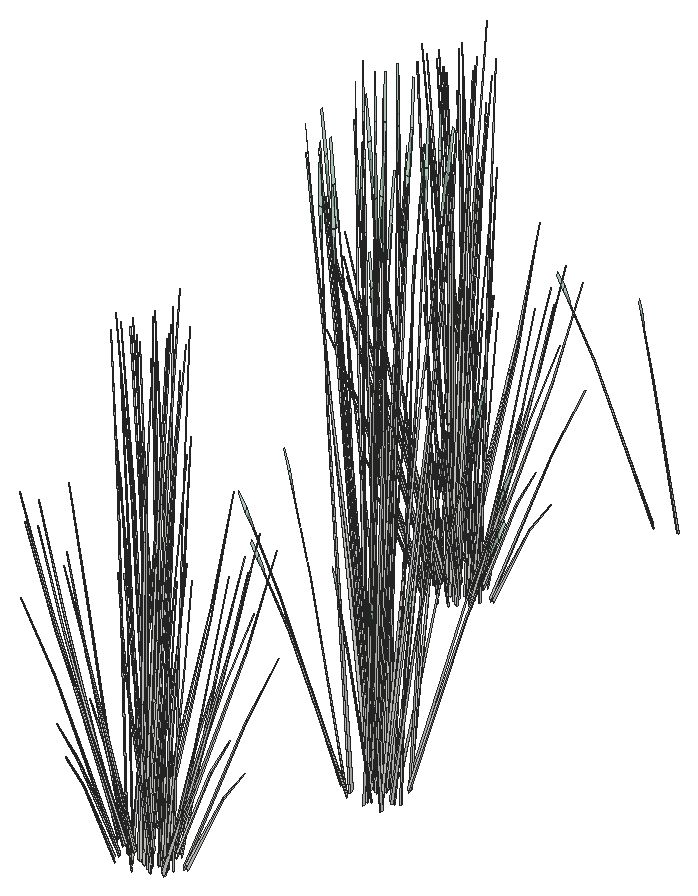
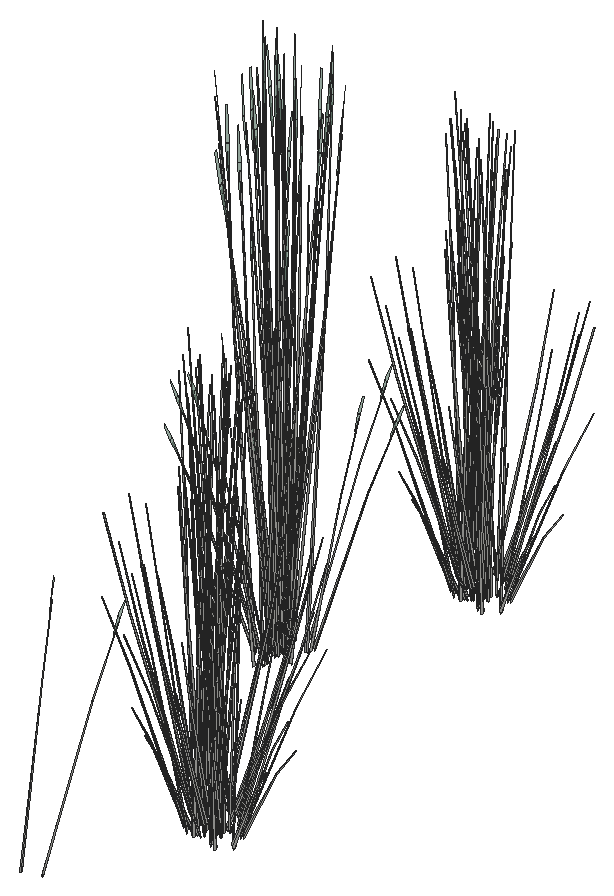
# SketchUp Ruby script. Lengths in inches.
U = 1.inch
M = Sketchup.active_model
def pt(a) = Geom::Point3d.new(a.map { |v| v * U })
def face(e, loops, mat)
  f = e.add_face(loops[0].map { |a| pt(a) })
  loops[1..].each { |l| e.add_face(l.map { |a| pt(a) }).erase! }
  f.material = f.back_material = mat if mat
  f
end
# faces: each face lists its corners as indices into pts; further lists are holes
def faces(e, pts, list, mat = nil) = list.each { |f| face(e, (f[0].is_a?(Array) ? f : [f]).map { |l| l.map { |i| pts[i] } }, mat) }
# xy, xz, yz: faces in a plane at the given z, y or x. An outline is a flat list of corners, or four numbers for a rectangle; further outlines are holes
def ring(l) = l.size == 4 ? [[l[0], l[1]], [l[2], l[1]], [l[2], l[3]], [l[0], l[3]]] : l.each_slice(2).to_a
def flat(e, list, mat, &to3) = list.each { |f| face(e, (f[0].is_a?(Array) ? f : [f]).map { |l| ring(l).map { |u, v| to3.(u, v) } }, mat) }
def xy(e, z, list, mat = nil) = flat(e, list, mat) { |x, y| [x, y, z] }
def xz(e, y, list, mat = nil) = flat(e, list, mat) { |x, z| [x, y, z] }
def yz(e, x, list, mat = nil) = flat(e, list, mat) { |y, z| [x, y, z] }
def lines(e, pts, list) = list.each { |a, b| e.add_line(pt(pts[a]), pt(pts[b])) }
# prism: a flat outline (further loops are holes) pulled along v
def prism(e, loops, v, mat = nil)
  f = face(e, loops, mat); d = Geom::Vector3d.new(v.map { |x| x * U })
  f.pushpull(f.normal.samedirection?(d) ? d.length : -d.length)
end
def box(e, o, s, mat = nil) = prism(e, [[o, [o[0] + s[0], o[1], o[2]], [o[0] + s[0], o[1] + s[1], o[2]], [o[0], o[1] + s[1], o[2]]]], [0, 0, s[2]], mat)
def at(x, y, z, deg = 0) = Geom::Transformation.translation(pt([x, y, z])) * Geom::Transformation.rotation(ORIGIN, Z_AXIS, deg.degrees)
def axes(o, x, y, z) = Geom::Transformation.new([*x, 0, *y, 0, *z, 0, *pt(o).to_a, 1])
def part(name) = M.definitions.add(name)
# library, detail: a bought-in or finely detailed component or shape, given as its bounding box
def library(name, o, s) = part(name).tap { |d| box(d.entities, o, s) }
def detail(e, o, s) = box(e.add_group.entities, o, s)
def put(e, d, t, mat = nil) = e.add_instance(d, t).tap { |i| i.material = mat if mat }
def group(e, t, mat = nil) = e.add_group.tap { |g| g.transformation = t; g.material = mat if mat }.entities
root = M.entities
M.materials.add("LightPink_Translucent").color = [175, 214, 192]
M.materials["LightPink_Translucent"].alpha = 0.75
c1 = part("blade")
p = [[2.15,0.21,22],[0,0.17,0],[0.09,0.45,0],[2.18,0.31,22],[2.29,0.31,22],[0.38,0.45,0],
  [2.48,0.24,33],[2.49,0.24,33],[2.48,0.22,33]]
faces(c1.entities,p,[[0,1,2,3],[4,5,2,3],[6,3,4,7],[8,0,3,6]])
c2 = part("blade with seeds\#1")
put(c2.entities,c1,at(0,0,0))
c3 = part("seeds")
p = [[0.3,-0.1,1.38],[-0.01,-0.03,1.59],[-0.01,-0.03,0.03],[0.14,-0.07,-0.07],[0.29,-0.03,3],[0.15,0.01,3.11]]
faces(c3.entities,p,[[0,1,2,3],[1,0,4,5]],"LightPink_Translucent")
c4 = part("blade with seeds")
put(c4.entities,c1,at(0,0,0))
put(c4.entities,c3,axes([2.4,0.25,30.99],[1.5799,-0.05474,1.17369],[-0.12525,1.92788,0.29478],[-0.07173,-0.02425,1.56792]))
put(root,c2,axes([494.86,352.5,140.9],[0.01294,-0.35246,-0.58282],[0.54471,0.02367,0.07033],[0.05748,-0.14932,0.82446]))
put(root,c2,axes([493.99,351.32,139.08],[0.06377,0.2222,0.94226],[-0.35378,-0.12306,0.69231],[0.03807,-0.11377,0.20754]))
put(root,c2,axes([493.69,352.14,140.65],[-0.48869,-0.09552,-0.41919],[0.16751,-0.3275,-0.3247],[-0.04481,-0.13186,0.80208]))
put(root,c2,axes([494.75,352.39,140.65],[-0.35588,-0.25603,-0.41919],[0.37594,-0.22422,-0.3247],[0.05415,-0.13008,0.80208]))
put(root,c2,axes([492.18,351.58,139.08],[0.25932,0.13262,0.94226],[-0.37767,0.07972,0.69231],[-0.08081,-0.10192,0.20754]))
put(root,c2,axes([492.8,352.29,140.9],[-0.4239,-0.18418,-0.58282],[0.30126,-0.32274,0.07033],[-0.15358,-0.10997,0.82446]))
put(root,c2,axes([492.6,352.3,140.65],[-0.49056,0.09058,-0.41919],[-0.08581,-0.34303,-0.3247],[-0.13176,-0.0983,0.80208]))
put(root,c2,axes([495.49,352.98,140.65],[-0.12771,-0.34793,-0.41919],[0.48364,-0.06086,-0.3247],[0.1386,-0.09345,0.80208]))
put(root,c2,axes([495.5,353.12,140.9],[0.25968,-0.30066,-0.58282],[0.45504,0.21367,0.07033],[0.15505,-0.10893,0.82446]))
put(root,c2,axes([495.875,352.84,138.9375],[-0.1776,-0.01129,1.17311],[-0.18194,-0.30276,-0.25229],[0.21818,-0.08565,0.50157]))
put(root,c2,axes([496.08,352.28,139.08],[-0.16559,0.19397,0.94226],[-0.14233,-0.26061,0.69231],[0.13676,-0.0653,0.20754]))
put(root,c2,axes([491.54,352.84,138.9375],[0.09706,0.10609,1.17311],[-0.22366,0.28837,-0.25229],[-0.22965,-0.06892,0.50157]))
put(root,c2,axes([491.9375,352.74,140.9],[-0.49695,-0.00917,-0.58282],[0.03338,-0.38634,0.07033],[-0.21053,-0.04077,0.82446]))
put(root,c2,axes([491.77,352.82,140.65],[-0.36098,0.25241,-0.41919],[-0.31614,-0.26664,-0.3247],[-0.18341,-0.0384,0.80208]))
put(root,c2,axes([493.38,353.64,138.81],[0.56014,0.18468,0.19741],[-0.26958,0.38374,0.41019],[0,-0.08846,1.31701]))
put(root,c2,axes([490.96,353.16,139.08],[0.31739,-0.02727,0.94226],[-0.20133,0.24024,0.69231],[-0.15684,-0.03604,0.20754]))
put(root,c2,axes([493.2,353.38,139.04],[-0.53984,0.02352,0.36702],[-0.04882,-0.39046,-0.17663],[0.09664,-0.03957,1.17838]))
put(root,c2,axes([491.81,353.66,138.85],[0,0.38104,0.40731],[-0.5562,0,0],[0,-0.08679,1.29208]))
put(root,c2,axes([493.18,353.52,138.75],[0.21614,0.42608,0.37535],[-0.61757,0.14817,0.14729],[0.00755,-0.07829,1.30318]))
put(root,c2,axes([495.71,353.75,140.65],[0.13468,-0.34661,-0.41919],[0.46175,0.1188,-0.3247],[0.18591,-0.03178,0.80208]))
put(root,c2,axes([494.71,352.54,138.85],[-0.46527,-0.19052,0.40731],[0.2781,-0.34163,0],[0.10597,0.04339,1.29208]))
put(root,c2,axes([493.07,353.85,139.04],[-0.2412,0.34335,0.36702],[-0.50118,-0.16524,-0.17663],[0,-0.07915,1.17838]))
put(root,c2,axes([493.67,353.28,138.75],[-0.41219,0.3458,0.37535],[-0.4897,-0.30525,0.14729],[0.09937,-0.03451,1.30318]))
put(root,c2,axes([492.95,352.71,138.84],[-0.14361,0.37869,0.14473],[-0.52552,-0.10717,0.28783],[0.09078,-0.00184,1.3159]))
put(root,c2,axes([495.625,353.875,140.9],[0.43684,-0.16829,-0.58282],[0.24345,0.34641,0.07033],[0.21107,-0.03935,0.82446]))
put(root,c2,axes([494.05,353.13,138.96],[0.0959,-0.34006,0.11878],[0.46856,0.05903,-0.33919],[0.08527,0.03492,1.03975]))
put(root,c2,axes([493.85,353.22,139.04],[-0.29864,-0.31983,0.36702],[0.45236,-0.22522,-0.17663],[0.09664,0.03957,1.17838]))
put(root,c2,axes([493.24,353.9375,138.75],[0.62833,0.08028,0.37535],[-0.12787,0.45342,0.14729],[-0.09182,-0.04378,1.30318]))
put(root,c2,axes([494.54,352.73,138.84],[-0.5342,0.10113,0.14473],[-0.13191,-0.37638,0.28783],[0.04764,0.05484,1.3159]))
put(root,c2,axes([492.9,354.66,138.84],[0.5342,-0.10113,0.14473],[0.13191,0.37638,0.28783],[-0.04764,-0.05484,1.3159]))
put(root,c2,axes([494.2,353.45,138.77],[-0.62833,-0.08028,0.4036],[0.12787,-0.45342,0.15838],[0.09182,0.04378,1.40127]))
put(root,c2,axes([493.39,354.26,138.96],[-0.0959,0.34006,0.11878],[-0.46856,-0.05903,-0.33919],[-0.08527,-0.03492,1.03975]))
put(root,c2,axes([494.37,353.82,138.63],[0.34702,0.24613,0],[-0.34702,0.24613,0],[0,0,1.38858]))
put(root,c2,axes([495.31,353.72,138.84],[-0.39059,-0.27756,0.14473],[0.39362,-0.26921,0.28783],[-0.04314,0.05668,1.3159]))
put(root,c2,axes([496.87,353.97,139.08],[-0.30716,0.06291,0.94226],[0.14458,-0.25998,0.69231],[0.16295,0.01779,0.20754]))
put(root,c2,axes([494.49,354.68,138.84],[0.14361,-0.37869,0.14473],[0.52552,0.10717,0.28783],[-0.09078,0.00184,1.3159]))
put(root,c2,axes([494.37,353.53,139.04],[0.2412,-0.34335,0.36702],[0.50118,0.16524,-0.17663],[0,0.07915,1.17838]))
put(root,c2,axes([492.73,354.85,138.85],[0.46527,0.19052,0.40731],[-0.2781,0.34163,0],[-0.10597,-0.04339,1.29208]))
put(root,c2,axes([491.42,353.57,140.65],[-0.13468,0.34661,-0.41919],[-0.46175,-0.1188,-0.3247],[-0.18591,0.03178,0.80208]))
put(root,c2,axes([495.63,353.73,138.85],[0,-0.38104,0.40731],[0.5562,0,0],[0,0.08679,1.29208]))
put(root,c2,axes([494.58,353.61,138.96],[0.46318,-0.11112,0.11878],[0.1622,0.31732,-0.33919],[0,0.06984,1.03975]))
put(root,c2,axes([494.24,354.01,139.04],[0.53984,-0.02352,0.36702],[0.04882,0.39046,-0.17663],[-0.09664,0.03957,1.17838]))
put(root,c2,axes([496.3,354.39,138.9375],[-0.11973,-0.09372,1.17311],[0.15578,-0.31002,-0.25229],[0.24224,0.042,0.50157]))
put(root,c2,axes([494.25,354.18,138.96],[0.36728,0.22894,0.11878],[-0.30636,0.25829,-0.33919],[-0.08527,0.03492,1.03975]))
put(root,c2,axes([495.2,354.58,140.9],[0.49695,0.00917,-0.58282],[-0.03338,0.38634,0.07033],[0.21053,0.04077,0.82446]))
put(root,c2,axes([494.64,354.88,138.85],[0.46527,-0.19052,0.40731],[0.2781,0.34163,0],[-0.10597,0.04339,1.29208]))
put(root,c2,axes([490.87,354.38,138.9375],[0.17277,0.03128,1.17311],[0.11135,0.3195,-0.25229],[-0.23468,0.05981,0.50157]))
put(root,c2,axes([490.51,355.05,139.08],[0.20718,-0.1727,0.94226],[0.08175,0.27339,0.69231],[-0.14972,0.04895,0.20754]))
put(root,c2,axes([495.16,354.87,139.08],[-0.27991,-0.10956,0.94226],[0.36143,-0.11132,0.69231],[0.09749,0.0943,0.20754]))
put(root,c2,axes([491.65,354.34,140.65],[0.12771,0.34793,-0.41919],[-0.48364,0.06086,-0.3247],[-0.1386,0.09345,0.80208]))
put(root,c2,axes([494.48,353.64,139.14],[-0.01358,-0.35877,1.15892],[0.61462,0.093,0.4907],[-0.14537,0.19631,1.09393]))
put(root,c2,axes([494.53,355.02,140.65],[0.49056,-0.09058,-0.41919],[0.08581,0.34303,-0.3247],[0.13176,0.0983,0.80208]))
put(root,c2,axes([495.21,355.37,139],[-0.31879,-0.01195,0.86186],[0.21053,-0.25381,0.47585],[0.12594,0.09017,0.67605]))
put(root,c2,axes([494.17,354.75,138.9375],[0.00877,-0.12631,1.17311],[0.41923,-0.14109,-0.25229],[0.12942,0.15118,0.50157]))
put(root,c2,axes([492.27,355.81,139.08],[-0.01287,-0.22657,0.94226],[0.32149,0.1616,0.69231],[-0.06323,0.10799,0.20754]))
put(root,c2,axes([493.44,355.18,140.65],[0.48869,0.09552,-0.41919],[-0.16751,0.3275,-0.3247],[0.04481,0.13186,0.80208]))
put(root,c2,axes([492,355.32,139.13],[0.45162,-0.06748,0.05338],[0.10383,0.27185,-0.708],[-0.02863,0.13761,0.63462]))
put(root,c2,axes([493.26,355.12,140.9],[0.23727,0.30983,-0.58282],[-0.48842,0.17267,0.07033],[0.05548,0.1497,0.82446]))
put(root,c2,axes([491.89,355.61,138.9375],[0.15688,-0.06011,1.17311],[0.38733,0.18125,-0.25229],[-0.11528,0.15683,0.50157]))
put(root,c4,axes([499.62,368.8,139.62],[-0.03656,0.1661,1.30132],[-0.37341,0.10705,-0.27986],[-0.0699,-0.22562,0.55638]))
put(root,c4,axes([501.43,369.44,139.62],[-0.12399,0.09331,1.30132],[-0.33702,-0.21502,-0.27986],[0.08055,-0.22079,0.55638]))
put(root,c4,axes([498.84,370.33,139.42],[-0.44625,-0.29882,0],[0.24886,-0.49993,-0.46963],[0.05668,-0.11386,1.48977]))
put(root,c4,axes([498.19,369.78,139.62],[0.07025,0.15082,1.30132],[-0.21183,0.37238,-0.27986],[-0.18329,-0.11083,0.55638]))
put(root,c4,axes([502.2,369.57,139.2],[-0.36364,-0.13787,-0.03542],[0.11186,-0.42434,-0.16061],[0.05948,-0.06443,0.52975]))
put(root,c4,axes([502.65,370.2,139.62],[-0.14568,-0.02894,1.30132],[-0.12195,-0.4231,-0.27986],[0.1883,-0.0989,0.55638]))
put(root,c4,axes([499.89,371.27,139.69],[-0.29566,-0.48255,-0.26477],[0.41776,-0.32089,-0.45502],[0.04243,-0.11906,1.45334]))
put(root,c4,axes([500.54,369.34,139.42],[0,-0.59763,0],[0.49772,0,-0.46963],[0.11336,0,1.48977]))
put(root,c4,axes([500.67,369.8,139.39],[-0.37441,-0.44456,0.27988],[0.37047,-0.44483,-0.33208],[0.10632,-0.01552,1.50045]))
put(root,c4,axes([499.76,371.8125,139.51],[0.35844,-0.4667,-0.22925],[0.40249,0.39271,0.50168],[-0.04193,-0.12567,1.53076]))
put(root,c4,axes([499.89,371.01,139.48],[0.5277,0.12668,-0.2132],[-0.09198,0.60063,0.46656],[0.07287,-0.10495,1.42361]))
put(root,c4,axes([499.76,371.23,139.65],[-0.39744,-0.0922,0.13176],[0.06899,-0.45047,-0.37626],[0.04081,-0.08198,1.15337]))
put(root,c4,axes([498.77,372.15,139.26],[0.44781,-0.29509,-0.04679],[0.24886,0.49993,0.46963],[-0.04264,-0.12319,1.48904]))
put(root,c4,axes([500.36,370.87,139.69],[0.21249,-0.53825,-0.26477],[0.44849,0.25917,-0.45502],[0.11011,-0.01692,1.45334]))
put(root,c4,axes([498.53,369.89,139.83],[0.07886,0.43418,0.05922],[-0.31771,0.09982,-0.78537],[-0.16083,-0.02753,0.70398]))
put(root,c4,axes([499.96,371.94,139.69],[-0.50815,0.05569,-0.26477],[-0.03072,-0.58006,-0.45502],[-0.06769,-0.10214,1.45334]))
put(root,c4,axes([502.66,371.21,139.2],[-0.25548,-0.33028,-0.03542],[0.27981,-0.30262,-0.16061],[0.07928,-0.02131,0.52975]))
put(root,c4,axes([500.14,371.08,139.41],[-0.09383,0.60408,0.41637],[-0.52992,-0.12294,0.16339],[0.05117,-0.08828,1.44559]))
put(root,c4,axes([499.22,371.41,139.26],[0.19993,-0.48183,0],[0.41543,0.23189,0],[0,0,1.48063]))
put(root,c4,axes([498.72,372.53,139.42],[-0.44625,0.29882,0],[-0.24886,-0.49993,-0.46963],[-0.05668,-0.11386,1.48977]))
put(root,c4,axes([499.86,372.05,139.65],[-0.26757,0.3531,0.13176],[-0.30187,-0.29453,-0.37626],[-0.04081,-0.08198,1.15337]))
put(root,c4,axes([500.1875,371.92,139.36],[0.3833,-0.44456,-0.05579],[0.38354,0.44483,0],[0.01339,-0.01552,1.5977]))
put(root,c4,axes([499,372.17,139.39],[-0.14475,0.59835,0.27988],[-0.51739,-0.14969,-0.33208],[-0.06475,-0.09903,1.50045]))
put(root,c4,axes([500.63,371.03,139.41],[-0.49797,0.2078,0.41637],[-0.17316,-0.59373,0.16339],[0.0915,0.00726,1.44559]))
put(root,c4,axes([499.4,371.52,139.27],[0.38394,-0.15594,0],[0.13445,0.4453,0],[0,0,1.40478]))
put(root,c4,axes([500.59,371.77,139.27],[0.51528,0,0],[0,0.59763,0],[0,0,1.63305]))
put(root,c4,axes([500.49,371.22,139.48],[-0.21584,0.53851,0.21899],[-0.44849,-0.25917,0.45502],[0.10338,0,1.46094]))
put(root,c4,axes([500.38,372.07,139.35],[-0.51503,0,-0.0513],[0,-0.59763,0],[-0.01619,0,1.63225]))
put(root,c4,axes([499.38,371.79,139.35],[-0.51161,0.2078,-0.05471],[-0.17927,-0.59373,0],[-0.01787,0.00726,1.56677]))
put(root,c4,axes([502.125,370.55,139.42],[0.44625,-0.29882,0],[0.24886,0.49993,-0.46963],[0.05668,0.11386,1.48977]))
put(root,c4,axes([500.06,373.5,139.27],[0.00356,-0.59734,-0.04529],[0.49772,0,0.45448],[-0.1133,-0.01877,1.441]))
put(root,c4,axes([500.91,371.49,139.41],[-0.40415,-0.39628,0.41637],[0.35675,-0.4708,0.16339],[0.04033,0.09554,1.44559]))
put(root,c4,axes([500.27,372.17,139.28],[-0.28765,0.33362,0],[-0.28765,-0.33362,0],[0,0,1.54032]))
put(root,c4,axes([499.22,371.96,139.27],[-0.19993,0.48183,0],[-0.41543,-0.23189,0],[0,0,1.59208]))
put(root,c4,axes([500.71,372.01,139.43],[0.09383,-0.60408,0.44771],[0.52992,0.12294,0.17569],[-0.05117,0.08828,1.5544]))
put(root,c4,axes([500.47,372.18,139.27],[0,0.53472,0],[-0.46104,0,0],[0,0,1.6235]))
put(root,c4,axes([500.89,371.14,139.69],[0.50815,-0.05569,-0.26477],[0.03072,0.58006,-0.45502],[0.06769,0.10214,1.45334]))
put(root,c4,axes([500.52,372.36,139.65],[0.12987,0.4453,0.13176],[-0.37086,0.15594,-0.37626],[-0.08162,0,1.15337]))
put(root,c4,axes([500.49,372.21,139.69],[-0.21249,0.53825,-0.26477],[-0.44849,-0.25917,-0.45502],[-0.11011,0.01692,1.45334]))
put(root,c4,axes([502.48,372.31,139.62],[-0.09014,-0.13585,1.30132],[0.15777,-0.40687,-0.27986],[0.19621,0.07542,0.55638]))
put(root,c4,axes([501.09,371.86,139.65],[0.39744,0.0922,0.13176],[-0.06899,0.45047,-0.37626],[-0.04081,0.08198,1.15337]))
put(root,c4,axes([499.45,372.11,139.25],[0.1511,0.50177,-0.1747],[-0.43526,0.17632,0.00007],[0.0167,0.05539,1.58246]))
put(root,c4,axes([499.1875,371.97,139.62],[0.14762,0.00843,1.30132],[0.1649,0.40305,-0.27986],[-0.17669,0.12442,0.55638]))
put(root,c4,axes([500.3125,373.74,139.43],[0,0.59763,0],[-0.49772,0,-0.46963],[-0.11336,0,1.48977]))
put(root,c4,axes([500.96,371.8125,139.69],[0.29566,0.48255,-0.26477],[-0.41776,0.32089,-0.45502],[-0.04243,0.11906,1.45334]))
put(root,c4,axes([501.22,370.59,138.72],[-0.17829,-0.47044,1.17325],[0.51157,-0.14973,0.45588],[-0.00851,0.28888,1.33444]))
put(root,c4,axes([502.01,372.75,139.43],[0.44625,0.29882,0],[-0.24886,0.49993,-0.46963],[-0.05668,0.11386,1.48977]))
put(root,c4,axes([500.625,374.49,139.32],[0.28477,-0.29631,-0.05904],[0.26092,0.32453,-0.26768],[0.01837,0.09195,0.88292]))
put(root,c4,axes([501.42,373.61,139.62],[0.01319,-0.17074,1.30132],[0.35385,-0.17492,-0.27986],[0.1001,0.20976,0.55638]))
put(root,c4,axes([500.25,373.93,139.07],[-0.05344,-0.30783,1.28841],[0.4254,-0.049,0.07375],[0.06439,0.2156,0.73315]))
put(root,c4,axes([499.62,374.02,139.62],[0.10953,-0.1151,1.30132],[0.36232,0.14976,-0.27986],[-0.04908,0.23288,0.55638]))
put(root,c2,axes([487.07,396.15,138.84],[-0.14131,0.07713,1.17311],[-0.4232,-0.13499,-0.25229],[0.07845,-0.16789,0.50157]))
put(root,c2,axes([486.43,396.41,140.8],[-0.23727,-0.30983,-0.58282],[0.48842,-0.17267,0.07033],[-0.05548,-0.1497,0.82446]))
put(root,c2,axes([484.89,396,138.84],[-0.0301,0.12465,1.17311],[-0.44009,0.10435,-0.25229],[-0.10287,-0.16111,0.50157]))
put(root,c2,axes([487.42,396.72,140.8],[0.01294,-0.35246,-0.58282],[0.54471,0.02367,0.07033],[0.05748,-0.14932,0.82446]))
put(root,c2,axes([486.55,395.53,138.99],[0.06377,0.2222,0.94226],[-0.35378,-0.12306,0.69231],[0.03807,-0.11377,0.20754]))
put(root,c2,axes([486.25,396.35,140.56],[-0.48869,-0.09552,-0.41919],[0.16751,-0.3275,-0.3247],[-0.04481,-0.13186,0.80208]))
put(root,c2,axes([487.31,396.6,140.56],[-0.35588,-0.25603,-0.41919],[0.37594,-0.22422,-0.3247],[0.05415,-0.13008,0.80208]))
put(root,c2,axes([484.73,395.8,138.99],[0.25932,0.13262,0.94226],[-0.37767,0.07972,0.69231],[-0.08081,-0.10192,0.20754]))
put(root,c2,axes([485.36,396.5,140.8],[-0.4239,-0.18418,-0.58282],[0.30126,-0.32274,0.07033],[-0.15358,-0.10997,0.82446]))
put(root,c2,axes([485.16,396.51,140.56],[-0.49056,0.09058,-0.41919],[-0.08581,-0.34303,-0.3247],[-0.13176,-0.0983,0.80208]))
put(root,c2,axes([488.05,397.1875,140.56],[-0.12771,-0.34793,-0.41919],[0.48364,-0.06086,-0.3247],[0.1386,-0.09345,0.80208]))
put(root,c2,axes([488.06,397.33,140.8],[0.25968,-0.30066,-0.58282],[0.45504,0.21367,0.07033],[0.15505,-0.10893,0.82446]))
put(root,c2,axes([488.43,397.05,138.84],[-0.1776,-0.01129,1.17311],[-0.18194,-0.30276,-0.25229],[0.21818,-0.08565,0.50157]))
put(root,c2,axes([488.64,396.5,138.99],[-0.16559,0.19397,0.94226],[-0.14233,-0.26061,0.69231],[0.13676,-0.0653,0.20754]))
put(root,c2,axes([484.09,397.05,138.84],[0.09706,0.10609,1.17311],[-0.22366,0.28837,-0.25229],[-0.22965,-0.06892,0.50157]))
put(root,c2,axes([484.5,396.96,140.8],[-0.49695,-0.00917,-0.58282],[0.03338,-0.38634,0.07033],[-0.21053,-0.04077,0.82446]))
put(root,c2,axes([484.33,397.03,140.56],[-0.36098,0.25241,-0.41919],[-0.31614,-0.26664,-0.3247],[-0.18341,-0.0384,0.80208]))
put(root,c2,axes([485.94,397.85,138.71],[0.56014,0.18468,0.19741],[-0.26958,0.38374,0.41019],[0,-0.08846,1.31701]))
put(root,c2,axes([483.52,397.37,138.99],[0.31739,-0.02727,0.94226],[-0.20133,0.24024,0.69231],[-0.15684,-0.03604,0.20754]))
put(root,c2,axes([485.76,397.59,138.95],[-0.53984,0.02352,0.36702],[-0.04882,-0.39046,-0.17663],[0.09664,-0.03957,1.17838]))
put(root,c2,axes([484.37,397.875,138.75],[0,0.38104,0.40731],[-0.5562,0,0],[0,-0.08679,1.29208]))
put(root,c2,axes([485.74,397.73,138.65],[0.21614,0.42608,0.37535],[-0.61757,0.14817,0.14729],[0.00755,-0.07829,1.30318]))
put(root,c2,axes([488.27,397.96,140.56],[0.13468,-0.34661,-0.41919],[0.46175,0.1188,-0.3247],[0.18591,-0.03178,0.80208]))
put(root,c2,axes([487.27,396.75,138.75],[-0.46527,-0.19052,0.40731],[0.2781,-0.34163,0],[0.10597,0.04339,1.29208]))
put(root,c2,axes([485.63,398.07,138.95],[-0.2412,0.34335,0.36702],[-0.50118,-0.16524,-0.17663],[0,-0.07915,1.17838]))
put(root,c2,axes([486.22,397.49,138.65],[-0.41219,0.3458,0.37535],[-0.4897,-0.30525,0.14729],[0.09937,-0.03451,1.30318]))
put(root,c2,axes([485.51,396.92,138.75],[-0.14361,0.37869,0.14473],[-0.52552,-0.10717,0.28783],[0.09078,-0.00184,1.3159]))
put(root,c2,axes([488.18,398.09,140.8],[0.43684,-0.16829,-0.58282],[0.24345,0.34641,0.07033],[0.21107,-0.03935,0.82446]))
put(root,c2,axes([486.61,397.34,138.86],[0.0959,-0.34006,0.11878],[0.46856,0.05903,-0.33919],[0.08527,0.03492,1.03975]))
put(root,c2,axes([486.41,397.43,138.95],[-0.29864,-0.31983,0.36702],[0.45236,-0.22522,-0.17663],[0.09664,0.03957,1.17838]))
put(root,c2,axes([485.8,398.15,138.65],[0.62833,0.08028,0.37535],[-0.12787,0.45342,0.14729],[-0.09182,-0.04378,1.30318]))
put(root,c2,axes([487.1,396.94,138.75],[-0.5342,0.10113,0.14473],[-0.13191,-0.37638,0.28783],[0.04764,0.05484,1.3159]))
put(root,c2,axes([485.46,398.875,138.75],[0.5342,-0.10113,0.14473],[0.13191,0.37638,0.28783],[-0.04764,-0.05484,1.3159]))
put(root,c2,axes([486.76,397.67,138.67],[-0.62833,-0.08028,0.4036],[0.12787,-0.45342,0.15838],[0.09182,0.04378,1.40127]))
put(root,c2,axes([485.95,398.47,138.86],[-0.0959,0.34006,0.11878],[-0.46856,-0.05903,-0.33919],[-0.08527,-0.03492,1.03975]))
put(root,c2,axes([487.87,397.93,138.75],[-0.39059,-0.27756,0.14473],[0.39362,-0.26921,0.28783],[-0.04314,0.05668,1.3159]))
put(root,c2,axes([484.96,397.57,139.46],[0.14131,-0.05512,1.45254],[0.04873,0.38487,0.11368],[-0.30608,0.05107,0.51915]))
put(root,c2,axes([489.43,398.18,138.99],[-0.30716,0.06291,0.94226],[0.14458,-0.25998,0.69231],[0.16295,0.01779,0.20754]))
put(root,c2,axes([487.05,398.89,138.75],[0.14361,-0.37869,0.14473],[0.52552,0.10717,0.28783],[-0.09078,0.00184,1.3159]))
put(root,c2,axes([486.92,397.75,138.95],[0.2412,-0.34335,0.36702],[0.50118,0.16524,-0.17663],[0,0.07915,1.17838]))
put(root,c2,axes([485.28,399.07,138.75],[0.46527,0.19052,0.40731],[-0.2781,0.34163,0],[-0.10597,-0.04339,1.29208]))
put(root,c2,axes([483.98,397.78,140.56],[-0.13468,0.34661,-0.41919],[-0.46175,-0.1188,-0.3247],[-0.18591,0.03178,0.80208]))
put(root,c2,axes([488.1875,397.9375,138.75],[0,-0.38104,0.40731],[0.5562,0,0],[0,0.08679,1.29208]))
put(root,c2,axes([487.13,397.83,138.86],[0.46318,-0.11112,0.11878],[0.1622,0.31732,-0.33919],[0,0.06984,1.03975]))
put(root,c2,axes([486.8,398.22,138.95],[0.53984,-0.02352,0.36702],[0.04882,0.39046,-0.17663],[-0.09664,0.03957,1.17838]))
put(root,c2,axes([488.85,398.6,138.84],[-0.11973,-0.09372,1.17311],[0.15578,-0.31002,-0.25229],[0.24224,0.042,0.50157]))
put(root,c2,axes([486.8,398.39,138.86],[0.36728,0.22894,0.11878],[-0.30636,0.25829,-0.33919],[-0.08527,0.03492,1.03975]))
put(root,c2,axes([487.76,398.79,140.8],[0.49695,0.00917,-0.58282],[-0.03338,0.38634,0.07033],[0.21053,0.04077,0.82446]))
put(root,c2,axes([487.2,399.1,138.75],[0.46527,-0.19052,0.40731],[0.2781,0.34163,0],[-0.10597,0.04339,1.29208]))
put(root,c2,axes([483.43,398.6,138.84],[0.17277,0.03128,1.17311],[0.11135,0.3195,-0.25229],[-0.23468,0.05981,0.50157]))
put(root,c2,axes([483.07,399.27,138.99],[0.20718,-0.1727,0.94226],[0.08175,0.27339,0.69231],[-0.14972,0.04895,0.20754]))
put(root,c2,axes([487.72,399.08,138.99],[-0.27991,-0.10956,0.94226],[0.36143,-0.11132,0.69231],[0.09749,0.0943,0.20754]))
put(root,c2,axes([484.21,398.56,140.56],[0.12771,0.34793,-0.41919],[-0.48364,0.06086,-0.3247],[-0.1386,0.09345,0.80208]))
put(root,c2,axes([487.04,397.85,139.05],[-0.01358,-0.35877,1.15892],[0.61462,0.093,0.4907],[-0.14537,0.19631,1.09393]))
put(root,c2,axes([487.09,399.23,140.56],[0.49056,-0.09058,-0.41919],[0.08581,0.34303,-0.3247],[0.13176,0.0983,0.80208]))
put(root,c2,axes([487.77,399.58,138.91],[-0.31879,-0.01195,0.86186],[0.21053,-0.25381,0.47585],[0.12594,0.09017,0.67605]))
put(root,c2,axes([486.73,398.97,138.84],[0.00877,-0.12631,1.17311],[0.41923,-0.14109,-0.25229],[0.12942,0.15118,0.50157]))
put(root,c2,axes([484.82,400.02,138.99],[-0.01287,-0.22657,0.94226],[0.32149,0.1616,0.69231],[-0.06323,0.10799,0.20754]))
put(root,c2,axes([486,399.39,140.56],[0.48869,0.09552,-0.41919],[-0.16751,0.3275,-0.3247],[0.04481,0.13186,0.80208]))
put(root,c2,axes([484.56,399.53,139.03],[0.45162,-0.06748,0.05338],[0.10383,0.27185,-0.708],[-0.02863,0.13761,0.63462]))
put(root,c2,axes([484.83,399.03,141.1],[-0.01294,0.35246,-0.64693],[-0.54471,-0.02367,0.07807],[-0.05748,0.14932,0.91515]))
put(root,c2,axes([485.82,399.33,140.8],[0.23727,0.30983,-0.58282],[-0.48842,0.17267,0.07033],[0.05548,0.1497,0.82446]))
put(root,c2,axes([484.45,399.82,138.84],[0.15688,-0.06011,1.17311],[0.38733,0.18125,-0.25229],[-0.11528,0.15683,0.50157]))
put(root,c4,axes([492.18,413.01,139.53],[-0.03656,0.1661,1.30132],[-0.37341,0.10705,-0.27986],[-0.0699,-0.22562,0.55638]))
put(root,c4,axes([493.98,413.66,139.53],[-0.12399,0.09331,1.30132],[-0.33702,-0.21502,-0.27986],[0.08055,-0.22079,0.55638]))
